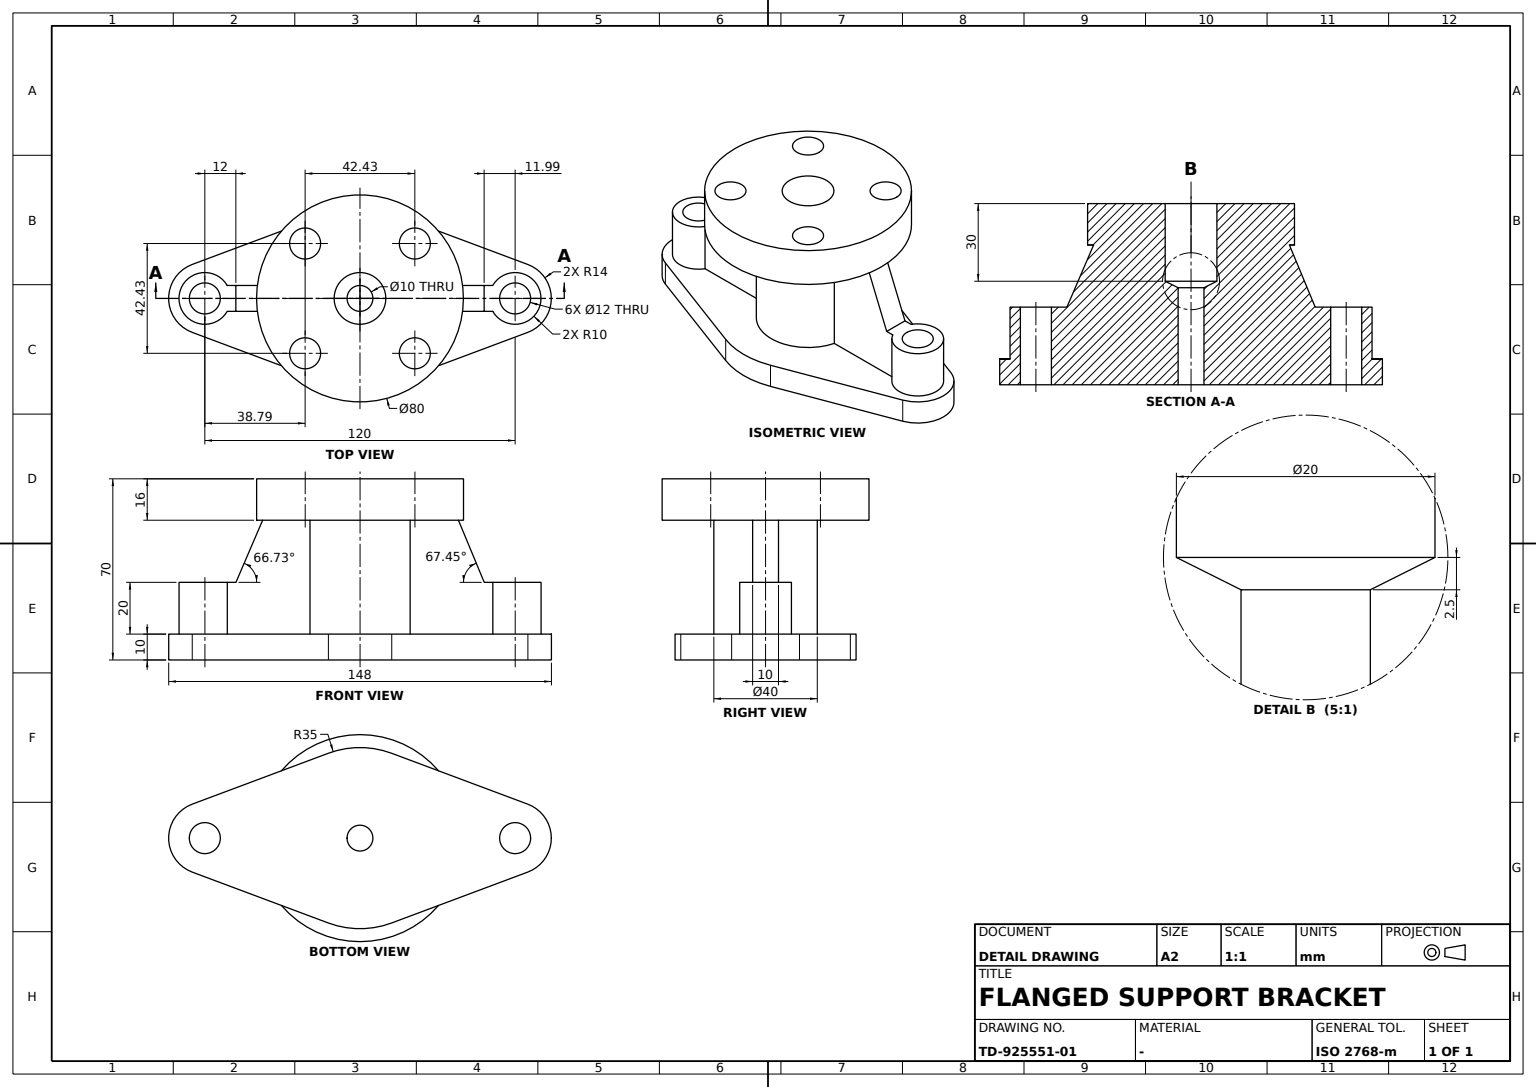
ISO-10303-21;
HEADER;
FILE_DESCRIPTION((''),'2;1');
FILE_NAME('','',(''),(''),'','','');
FILE_SCHEMA(('AUTOMOTIVE_DESIGN'));
ENDSEC;
DATA;
#1=APPLICATION_CONTEXT('');
#2=PRODUCT_CONTEXT('',#1,'mechanical');
#3=PRODUCT('','','',(#2));
#4=PRODUCT_DEFINITION_FORMATION('','',#3);
#5=PRODUCT_DEFINITION_CONTEXT('',#1,'design');
#6=PRODUCT_DEFINITION('','',#4,#5);
#7=PRODUCT_DEFINITION_SHAPE('','',#6);
#8=(LENGTH_UNIT()NAMED_UNIT(*)SI_UNIT(.MILLI.,.METRE.));
#9=(NAMED_UNIT(*)PLANE_ANGLE_UNIT()SI_UNIT($,.RADIAN.));
#10=(NAMED_UNIT(*)SI_UNIT($,.STERADIAN.)SOLID_ANGLE_UNIT());
#11=UNCERTAINTY_MEASURE_WITH_UNIT(LENGTH_MEASURE(1.E-05),#8,'distance_accuracy_value','');
#12=(GEOMETRIC_REPRESENTATION_CONTEXT(3)GLOBAL_UNCERTAINTY_ASSIGNED_CONTEXT((#11))GLOBAL_UNIT_ASSIGNED_CONTEXT((#8,#9,#10))REPRESENTATION_CONTEXT('',''));
#13=CARTESIAN_POINT('',(12.25,32.786239,10.));
#14=VERTEX_POINT('',#13);
#15=CARTESIAN_POINT('',(-12.25,32.786239,10.));
#16=VERTEX_POINT('',#15);
#17=CARTESIAN_POINT('',(0.,0.,10.));
#18=DIRECTION('',(0.,0.,1.));
#19=DIRECTION('',(1.,0.,0.));
#20=AXIS2_PLACEMENT_3D('',#17,#18,#19);
#21=CIRCLE('',#20,35.);
#22=EDGE_CURVE('',#14,#16,#21,.T.);
#23=ORIENTED_EDGE('',*,*,#22,.F.);
#24=CARTESIAN_POINT('',(12.25,32.786239,0.));
#25=VERTEX_POINT('',#24);
#26=CARTESIAN_POINT('',(12.25,32.786239,5.));
#27=VECTOR('',#18,1000.);
#28=LINE('',#26,#27);
#29=EDGE_CURVE('',#25,#14,#28,.T.);
#30=ORIENTED_EDGE('',*,*,#29,.F.);
#31=CARTESIAN_POINT('',(-12.25,32.786239,0.));
#32=VERTEX_POINT('',#31);
#33=CARTESIAN_POINT('',(0.,0.,0.));
#34=AXIS2_PLACEMENT_3D('',#33,#18,#19);
#35=CIRCLE('',#34,35.);
#36=EDGE_CURVE('',#25,#32,#35,.T.);
#37=ORIENTED_EDGE('',*,*,#36,.T.);
#38=CARTESIAN_POINT('',(-12.25,32.786239,5.));
#39=LINE('',#38,#27);
#40=EDGE_CURVE('',#32,#16,#39,.T.);
#41=ORIENTED_EDGE('',*,*,#40,.T.);
#42=EDGE_LOOP('',(#23,#30,#37,#41));
#43=FACE_OUTER_BOUND('',#42,.T.);
#44=CARTESIAN_POINT('',(0.,0.,5.));
#45=DIRECTION('',(0.,0.,-1.));
#46=AXIS2_PLACEMENT_3D('',#44,#45,#19);
#47=CYLINDRICAL_SURFACE('',#46,35.);
#48=ADVANCED_FACE('',(#43),#47,.T.);
#49=CARTESIAN_POINT('',(-37.677164,5.,54.));
#50=VERTEX_POINT('',#49);
#51=CARTESIAN_POINT('',(-19.364917,5.,54.));
#52=VERTEX_POINT('',#51);
#53=CARTESIAN_POINT('',(-28.52104,5.,54.));
#54=VECTOR('',#19,1000.);
#55=LINE('',#53,#54);
#56=EDGE_CURVE('',#50,#52,#55,.T.);
#57=ORIENTED_EDGE('',*,*,#56,.F.);
#58=CARTESIAN_POINT('',(-37.677164,-5.,54.));
#59=VERTEX_POINT('',#58);
#60=CARTESIAN_POINT('',(-37.677164,0.,54.));
#61=DIRECTION('',(0.,-1.,0.));
#62=VECTOR('',#61,1000.);
#63=LINE('',#60,#62);
#64=EDGE_CURVE('',#50,#59,#63,.T.);
#65=ORIENTED_EDGE('',*,*,#64,.T.);
#66=CARTESIAN_POINT('',(-19.364917,-5.,54.));
#67=VERTEX_POINT('',#66);
#68=CARTESIAN_POINT('',(-28.52104,-5.,54.));
#69=LINE('',#68,#54);
#70=EDGE_CURVE('',#59,#67,#69,.T.);
#71=ORIENTED_EDGE('',*,*,#70,.T.);
#72=CARTESIAN_POINT('',(19.364917,-5.,54.));
#73=VERTEX_POINT('',#72);
#74=CARTESIAN_POINT('',(0.,0.,54.));
#75=AXIS2_PLACEMENT_3D('',#74,#18,#19);
#76=CIRCLE('',#75,20.);
#77=EDGE_CURVE('',#67,#73,#76,.T.);
#78=ORIENTED_EDGE('',*,*,#77,.T.);
#79=CARTESIAN_POINT('',(38.044305,-5.,54.));
#80=VERTEX_POINT('',#79);
#81=CARTESIAN_POINT('',(28.704611,-5.,54.));
#82=LINE('',#81,#54);
#83=EDGE_CURVE('',#73,#80,#82,.T.);
#84=ORIENTED_EDGE('',*,*,#83,.T.);
#85=CARTESIAN_POINT('',(38.044305,5.,54.));
#86=VERTEX_POINT('',#85);
#87=CARTESIAN_POINT('',(38.044305,0.,54.));
#88=LINE('',#87,#62);
#89=EDGE_CURVE('',#86,#80,#88,.T.);
#90=ORIENTED_EDGE('',*,*,#89,.F.);
#91=CARTESIAN_POINT('',(19.364917,5.,54.));
#92=VERTEX_POINT('',#91);
#93=CARTESIAN_POINT('',(28.704611,5.,54.));
#94=LINE('',#93,#54);
#95=EDGE_CURVE('',#92,#86,#94,.T.);
#96=ORIENTED_EDGE('',*,*,#95,.F.);
#97=EDGE_CURVE('',#92,#52,#76,.T.);
#98=ORIENTED_EDGE('',*,*,#97,.T.);
#99=EDGE_LOOP('',(#57,#65,#71,#78,#84,#90,#96,#98));
#100=FACE_BOUND('',#99,.T.);
#101=CARTESIAN_POINT('',(-15.213203,-21.213203,54.));
#102=VERTEX_POINT('',#101);
#103=CARTESIAN_POINT('',(-27.213203,-21.213203,54.));
#104=VERTEX_POINT('',#103);
#105=CARTESIAN_POINT('',(-21.213203,-21.213203,54.));
#106=AXIS2_PLACEMENT_3D('',#105,#18,#19);
#107=CIRCLE('',#106,6.);
#108=EDGE_CURVE('',#102,#104,#107,.T.);
#109=ORIENTED_EDGE('',*,*,#108,.T.);
#110=EDGE_CURVE('',#104,#102,#107,.T.);
#111=ORIENTED_EDGE('',*,*,#110,.T.);
#112=EDGE_LOOP('',(#109,#111));
#113=FACE_BOUND('',#112,.T.);
#114=CARTESIAN_POINT('',(40.,0.,54.));
#115=VERTEX_POINT('',#114);
#116=CARTESIAN_POINT('',(-40.,0.,54.));
#117=VERTEX_POINT('',#116);
#118=CIRCLE('',#75,40.);
#119=EDGE_CURVE('',#115,#117,#118,.T.);
#120=ORIENTED_EDGE('',*,*,#119,.F.);
#121=EDGE_CURVE('',#117,#115,#118,.T.);
#122=ORIENTED_EDGE('',*,*,#121,.F.);
#123=EDGE_LOOP('',(#120,#122));
#124=FACE_OUTER_BOUND('',#123,.T.);
#125=CARTESIAN_POINT('',(15.213203,21.213203,54.));
#126=VERTEX_POINT('',#125);
#127=CARTESIAN_POINT('',(27.213203,21.213203,54.));
#128=VERTEX_POINT('',#127);
#129=CARTESIAN_POINT('',(21.213203,21.213203,54.));
#130=AXIS2_PLACEMENT_3D('',#129,#18,#19);
#131=CIRCLE('',#130,6.);
#132=EDGE_CURVE('',#126,#128,#131,.T.);
#133=ORIENTED_EDGE('',*,*,#132,.T.);
#134=EDGE_CURVE('',#128,#126,#131,.T.);
#135=ORIENTED_EDGE('',*,*,#134,.T.);
#136=EDGE_LOOP('',(#133,#135));
#137=FACE_BOUND('',#136,.T.);
#138=CARTESIAN_POINT('',(-27.213203,21.213203,54.));
#139=VERTEX_POINT('',#138);
#140=CARTESIAN_POINT('',(-15.213203,21.213203,54.));
#141=VERTEX_POINT('',#140);
#142=CARTESIAN_POINT('',(-21.213203,21.213203,54.));
#143=AXIS2_PLACEMENT_3D('',#142,#18,#19);
#144=CIRCLE('',#143,6.);
#145=EDGE_CURVE('',#139,#141,#144,.T.);
#146=ORIENTED_EDGE('',*,*,#145,.T.);
#147=EDGE_CURVE('',#141,#139,#144,.T.);
#148=ORIENTED_EDGE('',*,*,#147,.T.);
#149=EDGE_LOOP('',(#146,#148));
#150=FACE_BOUND('',#149,.T.);
#151=CARTESIAN_POINT('',(27.213203,-21.213203,54.));
#152=VERTEX_POINT('',#151);
#153=CARTESIAN_POINT('',(15.213203,-21.213203,54.));
#154=VERTEX_POINT('',#153);
#155=CARTESIAN_POINT('',(21.213203,-21.213203,54.));
#156=AXIS2_PLACEMENT_3D('',#155,#18,#19);
#157=CIRCLE('',#156,6.);
#158=EDGE_CURVE('',#152,#154,#157,.T.);
#159=ORIENTED_EDGE('',*,*,#158,.T.);
#160=EDGE_CURVE('',#154,#152,#157,.T.);
#161=ORIENTED_EDGE('',*,*,#160,.T.);
#162=EDGE_LOOP('',(#159,#161));
#163=FACE_BOUND('',#162,.T.);
#164=PLANE('',#75);
#165=ADVANCED_FACE('',(#100,#113,#124,#137,#150,#163),#164,.F.);
#166=CARTESIAN_POINT('',(64.9,13.114496,0.));
#167=VERTEX_POINT('',#166);
#168=CARTESIAN_POINT('',(64.9,13.114496,10.));
#169=VERTEX_POINT('',#168);
#170=CARTESIAN_POINT('',(64.9,13.114496,5.));
#171=LINE('',#170,#27);
#172=EDGE_CURVE('',#167,#169,#171,.T.);
#173=ORIENTED_EDGE('',*,*,#172,.T.);
#174=CARTESIAN_POINT('',(74.,0.,10.));
#175=VERTEX_POINT('',#174);
#176=CARTESIAN_POINT('',(60.,0.,10.));
#177=AXIS2_PLACEMENT_3D('',#176,#18,#19);
#178=CIRCLE('',#177,14.);
#179=EDGE_CURVE('',#175,#169,#178,.T.);
#180=ORIENTED_EDGE('',*,*,#179,.F.);
#181=CARTESIAN_POINT('',(74.,0.,0.));
#182=VERTEX_POINT('',#181);
#183=CARTESIAN_POINT('',(74.,0.,5.));
#184=VECTOR('',#45,1000.);
#185=LINE('',#183,#184);
#186=EDGE_CURVE('',#175,#182,#185,.T.);
#187=ORIENTED_EDGE('',*,*,#186,.T.);
#188=CARTESIAN_POINT('',(60.,0.,0.));
#189=AXIS2_PLACEMENT_3D('',#188,#18,#19);
#190=CIRCLE('',#189,14.);
#191=EDGE_CURVE('',#182,#167,#190,.T.);
#192=ORIENTED_EDGE('',*,*,#191,.T.);
#193=EDGE_LOOP('',(#173,#180,#187,#192));
#194=FACE_OUTER_BOUND('',#193,.T.);
#195=CARTESIAN_POINT('',(60.,0.,5.));
#196=AXIS2_PLACEMENT_3D('',#195,#45,#19);
#197=CYLINDRICAL_SURFACE('',#196,14.);
#198=ADVANCED_FACE('',(#194),#197,.T.);
#199=ORIENTED_EDGE('',*,*,#29,.T.);
#200=CARTESIAN_POINT('',(38.575,22.950368,10.));
#201=DIRECTION('',(-0.9367497,0.35,0.));
#202=VECTOR('',#201,1000.);
#203=LINE('',#200,#202);
#204=EDGE_CURVE('',#169,#14,#203,.T.);
#205=ORIENTED_EDGE('',*,*,#204,.F.);
#206=ORIENTED_EDGE('',*,*,#172,.F.);
#207=CARTESIAN_POINT('',(38.575,22.950368,0.));
#208=LINE('',#207,#202);
#209=EDGE_CURVE('',#167,#25,#208,.T.);
#210=ORIENTED_EDGE('',*,*,#209,.T.);
#211=EDGE_LOOP('',(#199,#205,#206,#210));
#212=FACE_OUTER_BOUND('',#211,.T.);
#213=DIRECTION('',(-0.35,-0.9367497,0.));
#214=DIRECTION('',(0.9367497,-0.35,0.));
#215=AXIS2_PLACEMENT_3D('',#24,#213,#214);
#216=PLANE('',#215);
#217=ADVANCED_FACE('',(#212),#216,.F.);
#218=CARTESIAN_POINT('',(-12.25,-32.786239,0.));
#219=VERTEX_POINT('',#218);
#220=CARTESIAN_POINT('',(-12.25,-32.786239,10.));
#221=VERTEX_POINT('',#220);
#222=CARTESIAN_POINT('',(-12.25,-32.786239,5.));
#223=LINE('',#222,#27);
#224=EDGE_CURVE('',#219,#221,#223,.T.);
#225=ORIENTED_EDGE('',*,*,#224,.F.);
#226=CARTESIAN_POINT('',(12.25,-32.786239,0.));
#227=VERTEX_POINT('',#226);
#228=EDGE_CURVE('',#219,#227,#35,.T.);
#229=ORIENTED_EDGE('',*,*,#228,.T.);
#230=CARTESIAN_POINT('',(12.25,-32.786239,10.));
#231=VERTEX_POINT('',#230);
#232=CARTESIAN_POINT('',(12.25,-32.786239,5.));
#233=LINE('',#232,#27);
#234=EDGE_CURVE('',#227,#231,#233,.T.);
#235=ORIENTED_EDGE('',*,*,#234,.T.);
#236=EDGE_CURVE('',#221,#231,#21,.T.);
#237=ORIENTED_EDGE('',*,*,#236,.F.);
#238=EDGE_LOOP('',(#225,#229,#235,#237));
#239=FACE_OUTER_BOUND('',#238,.T.);
#240=ADVANCED_FACE('',(#239),#47,.T.);
#241=CARTESIAN_POINT('',(-64.9,-13.114496,10.));
#242=VERTEX_POINT('',#241);
#243=CARTESIAN_POINT('',(-38.575,-22.950368,10.));
#244=VECTOR('',#214,1000.);
#245=LINE('',#243,#244);
#246=EDGE_CURVE('',#242,#221,#245,.T.);
#247=ORIENTED_EDGE('',*,*,#246,.F.);
#248=CARTESIAN_POINT('',(-64.9,-13.114496,0.));
#249=VERTEX_POINT('',#248);
#250=CARTESIAN_POINT('',(-64.9,-13.114496,5.));
#251=LINE('',#250,#27);
#252=EDGE_CURVE('',#249,#242,#251,.T.);
#253=ORIENTED_EDGE('',*,*,#252,.F.);
#254=CARTESIAN_POINT('',(-38.575,-22.950368,0.));
#255=LINE('',#254,#244);
#256=EDGE_CURVE('',#249,#219,#255,.T.);
#257=ORIENTED_EDGE('',*,*,#256,.T.);
#258=ORIENTED_EDGE('',*,*,#224,.T.);
#259=EDGE_LOOP('',(#247,#253,#257,#258));
#260=FACE_OUTER_BOUND('',#259,.T.);
#261=AXIS2_PLACEMENT_3D('',#248,#213,#214);
#262=PLANE('',#261);
#263=ADVANCED_FACE('',(#260),#262,.T.);
#264=CARTESIAN_POINT('',(51.339746,5.,10.));
#265=VERTEX_POINT('',#264);
#266=CARTESIAN_POINT('',(51.339746,5.,30.));
#267=VERTEX_POINT('',#266);
#268=CARTESIAN_POINT('',(51.339746,5.,20.));
#269=LINE('',#268,#27);
#270=EDGE_CURVE('',#265,#267,#269,.T.);
#271=ORIENTED_EDGE('',*,*,#270,.T.);
#272=CARTESIAN_POINT('',(70.,0.,30.));
#273=VERTEX_POINT('',#272);
#274=CARTESIAN_POINT('',(60.,0.,30.));
#275=AXIS2_PLACEMENT_3D('',#274,#18,#19);
#276=CIRCLE('',#275,10.);
#277=EDGE_CURVE('',#273,#267,#276,.T.);
#278=ORIENTED_EDGE('',*,*,#277,.F.);
#279=CARTESIAN_POINT('',(70.,0.,10.));
#280=VERTEX_POINT('',#279);
#281=CARTESIAN_POINT('',(70.,0.,20.));
#282=LINE('',#281,#27);
#283=EDGE_CURVE('',#280,#273,#282,.T.);
#284=ORIENTED_EDGE('',*,*,#283,.F.);
#285=CIRCLE('',#177,10.);
#286=EDGE_CURVE('',#280,#265,#285,.T.);
#287=ORIENTED_EDGE('',*,*,#286,.T.);
#288=EDGE_LOOP('',(#271,#278,#284,#287));
#289=FACE_OUTER_BOUND('',#288,.T.);
#290=CARTESIAN_POINT('',(60.,0.,20.));
#291=AXIS2_PLACEMENT_3D('',#290,#45,#19);
#292=CYLINDRICAL_SURFACE('',#291,10.);
#293=ADVANCED_FACE('',(#289),#292,.T.);
#294=CARTESIAN_POINT('',(-64.9,13.114496,0.));
#295=VERTEX_POINT('',#294);
#296=CARTESIAN_POINT('',(-64.9,13.114496,10.));
#297=VERTEX_POINT('',#296);
#298=CARTESIAN_POINT('',(-64.9,13.114496,5.));
#299=LINE('',#298,#27);
#300=EDGE_CURVE('',#295,#297,#299,.T.);
#301=ORIENTED_EDGE('',*,*,#300,.F.);
#302=CARTESIAN_POINT('',(-60.,0.,0.));
#303=AXIS2_PLACEMENT_3D('',#302,#18,#19);
#304=CIRCLE('',#303,14.);
#305=EDGE_CURVE('',#295,#249,#304,.T.);
#306=ORIENTED_EDGE('',*,*,#305,.T.);
#307=ORIENTED_EDGE('',*,*,#252,.T.);
#308=CARTESIAN_POINT('',(-60.,0.,10.));
#309=AXIS2_PLACEMENT_3D('',#308,#18,#19);
#310=CIRCLE('',#309,14.);
#311=EDGE_CURVE('',#297,#242,#310,.T.);
#312=ORIENTED_EDGE('',*,*,#311,.F.);
#313=EDGE_LOOP('',(#301,#306,#307,#312));
#314=FACE_OUTER_BOUND('',#313,.T.);
#315=CARTESIAN_POINT('',(-60.,0.,5.));
#316=AXIS2_PLACEMENT_3D('',#315,#45,#19);
#317=CYLINDRICAL_SURFACE('',#316,14.);
#318=ADVANCED_FACE('',(#314),#317,.T.);
#319=CARTESIAN_POINT('',(50.277016,-5.,30.));
#320=VERTEX_POINT('',#319);
#321=CARTESIAN_POINT('',(50.277016,5.,30.));
#322=VERTEX_POINT('',#321);
#323=CARTESIAN_POINT('',(50.277016,0.,30.));
#324=DIRECTION('',(0.,1.,0.));
#325=VECTOR('',#324,1000.);
#326=LINE('',#323,#325);
#327=EDGE_CURVE('',#320,#322,#326,.T.);
#328=ORIENTED_EDGE('',*,*,#327,.T.);
#329=CARTESIAN_POINT('',(48.011559,5.,30.));
#330=VERTEX_POINT('',#329);
#331=CARTESIAN_POINT('',(49.144287,5.,30.));
#332=DIRECTION('',(-1.,0.,0.));
#333=VECTOR('',#332,1000.);
#334=LINE('',#331,#333);
#335=EDGE_CURVE('',#322,#330,#334,.T.);
#336=ORIENTED_EDGE('',*,*,#335,.T.);
#337=CARTESIAN_POINT('',(48.011559,-5.,30.));
#338=VERTEX_POINT('',#337);
#339=CARTESIAN_POINT('',(48.011559,0.,30.));
#340=LINE('',#339,#325);
#341=EDGE_CURVE('',#338,#330,#340,.T.);
#342=ORIENTED_EDGE('',*,*,#341,.F.);
#343=CARTESIAN_POINT('',(49.144287,-5.,30.));
#344=LINE('',#343,#333);
#345=EDGE_CURVE('',#320,#338,#344,.T.);
#346=ORIENTED_EDGE('',*,*,#345,.F.);
#347=EDGE_LOOP('',(#328,#336,#342,#346));
#348=FACE_OUTER_BOUND('',#347,.T.);
#349=CARTESIAN_POINT('',(0.,0.,30.));
#350=AXIS2_PLACEMENT_3D('',#349,#18,#19);
#351=PLANE('',#350);
#352=ADVANCED_FACE('',(#348),#351,.T.);
#353=ORIENTED_EDGE('',*,*,#121,.T.);
#354=CARTESIAN_POINT('',(40.,0.,70.));
#355=VERTEX_POINT('',#354);
#356=CARTESIAN_POINT('',(40.,0.,62.));
#357=LINE('',#356,#27);
#358=EDGE_CURVE('',#115,#355,#357,.T.);
#359=ORIENTED_EDGE('',*,*,#358,.T.);
#360=CARTESIAN_POINT('',(-40.,0.,70.));
#361=VERTEX_POINT('',#360);
#362=CARTESIAN_POINT('',(0.,0.,70.));
#363=AXIS2_PLACEMENT_3D('',#362,#18,#19);
#364=CIRCLE('',#363,40.);
#365=EDGE_CURVE('',#361,#355,#364,.T.);
#366=ORIENTED_EDGE('',*,*,#365,.F.);
#367=CARTESIAN_POINT('',(-40.,0.,62.));
#368=LINE('',#367,#27);
#369=EDGE_CURVE('',#117,#361,#368,.T.);
#370=ORIENTED_EDGE('',*,*,#369,.F.);
#371=EDGE_LOOP('',(#353,#359,#366,#370));
#372=FACE_OUTER_BOUND('',#371,.T.);
#373=CARTESIAN_POINT('',(0.,0.,62.));
#374=AXIS2_PLACEMENT_3D('',#373,#45,#19);
#375=CYLINDRICAL_SURFACE('',#374,40.);
#376=ADVANCED_FACE('',(#372),#375,.T.);
#377=CARTESIAN_POINT('',(-15.213203,-21.213203,70.));
#378=VERTEX_POINT('',#377);
#379=CARTESIAN_POINT('',(-15.213203,-21.213203,62.));
#380=LINE('',#379,#184);
#381=EDGE_CURVE('',#378,#102,#380,.T.);
#382=ORIENTED_EDGE('',*,*,#381,.T.);
#383=ORIENTED_EDGE('',*,*,#110,.F.);
#384=CARTESIAN_POINT('',(-27.213203,-21.213203,70.));
#385=VERTEX_POINT('',#384);
#386=CARTESIAN_POINT('',(-27.213203,-21.213203,62.));
#387=LINE('',#386,#184);
#388=EDGE_CURVE('',#385,#104,#387,.T.);
#389=ORIENTED_EDGE('',*,*,#388,.F.);
#390=CARTESIAN_POINT('',(-21.213203,-21.213203,70.));
#391=AXIS2_PLACEMENT_3D('',#390,#18,#19);
#392=CIRCLE('',#391,6.);
#393=EDGE_CURVE('',#385,#378,#392,.T.);
#394=ORIENTED_EDGE('',*,*,#393,.T.);
#395=EDGE_LOOP('',(#382,#383,#389,#394));
#396=FACE_OUTER_BOUND('',#395,.T.);
#397=CARTESIAN_POINT('',(-21.213203,-21.213203,62.));
#398=AXIS2_PLACEMENT_3D('',#397,#45,#19);
#399=CYLINDRICAL_SURFACE('',#398,6.);
#400=ADVANCED_FACE('',(#396),#399,.F.);
#401=CARTESIAN_POINT('',(5.,0.,37.5));
#402=VERTEX_POINT('',#401);
#403=CARTESIAN_POINT('',(10.,0.,40.));
#404=VERTEX_POINT('',#403);
#405=CARTESIAN_POINT('',(7.5,0.,38.75));
#406=DIRECTION('',(0.894427191,0.,0.447213595));
#407=VECTOR('',#406,1000.);
#408=LINE('',#405,#407);
#409=EDGE_CURVE('',#402,#404,#408,.T.);
#410=ORIENTED_EDGE('',*,*,#409,.F.);
#411=CARTESIAN_POINT('',(-5.,0.,37.5));
#412=VERTEX_POINT('',#411);
#413=CARTESIAN_POINT('',(0.,0.,37.5));
#414=AXIS2_PLACEMENT_3D('',#413,#18,#19);
#415=CIRCLE('',#414,5.);
#416=EDGE_CURVE('',#412,#402,#415,.T.);
#417=ORIENTED_EDGE('',*,*,#416,.F.);
#418=CARTESIAN_POINT('',(-10.,0.,40.));
#419=VERTEX_POINT('',#418);
#420=CARTESIAN_POINT('',(-7.5,0.,38.75));
#421=DIRECTION('',(-0.894427191,0.,0.447213595));
#422=VECTOR('',#421,1000.);
#423=LINE('',#420,#422);
#424=EDGE_CURVE('',#412,#419,#423,.T.);
#425=ORIENTED_EDGE('',*,*,#424,.T.);
#426=CARTESIAN_POINT('',(0.,0.,40.));
#427=AXIS2_PLACEMENT_3D('',#426,#45,#19);
#428=CIRCLE('',#427,10.);
#429=EDGE_CURVE('',#404,#419,#428,.T.);
#430=ORIENTED_EDGE('',*,*,#429,.F.);
#431=EDGE_LOOP('',(#410,#417,#425,#430));
#432=FACE_OUTER_BOUND('',#431,.T.);
#433=CONICAL_SURFACE('',#414,5.,1.107148718);
#434=ADVANCED_FACE('',(#432),#433,.F.);
#435=CARTESIAN_POINT('',(64.9,-13.114496,0.));
#436=VERTEX_POINT('',#435);
#437=CARTESIAN_POINT('',(38.575,-22.950368,0.));
#438=DIRECTION('',(0.9367497,0.35,0.));
#439=VECTOR('',#438,1000.);
#440=LINE('',#437,#439);
#441=EDGE_CURVE('',#227,#436,#440,.T.);
#442=ORIENTED_EDGE('',*,*,#441,.T.);
#443=CARTESIAN_POINT('',(64.9,-13.114496,10.));
#444=VERTEX_POINT('',#443);
#445=CARTESIAN_POINT('',(64.9,-13.114496,5.));
#446=LINE('',#445,#27);
#447=EDGE_CURVE('',#436,#444,#446,.T.);
#448=ORIENTED_EDGE('',*,*,#447,.T.);
#449=CARTESIAN_POINT('',(38.575,-22.950368,10.));
#450=LINE('',#449,#439);
#451=EDGE_CURVE('',#231,#444,#450,.T.);
#452=ORIENTED_EDGE('',*,*,#451,.F.);
#453=ORIENTED_EDGE('',*,*,#234,.F.);
#454=EDGE_LOOP('',(#442,#448,#452,#453));
#455=FACE_OUTER_BOUND('',#454,.T.);
#456=DIRECTION('',(0.35,-0.9367497,0.));
#457=AXIS2_PLACEMENT_3D('',#226,#456,#438);
#458=PLANE('',#457);
#459=ADVANCED_FACE('',(#455),#458,.T.);
#460=CARTESIAN_POINT('',(-70.,0.,10.));
#461=VERTEX_POINT('',#460);
#462=CARTESIAN_POINT('',(-51.339746,-5.,10.));
#463=VERTEX_POINT('',#462);
#464=CIRCLE('',#309,10.);
#465=EDGE_CURVE('',#461,#463,#464,.T.);
#466=ORIENTED_EDGE('',*,*,#465,.T.);
#467=CARTESIAN_POINT('',(-51.339746,-5.,30.));
#468=VERTEX_POINT('',#467);
#469=CARTESIAN_POINT('',(-51.339746,-5.,20.));
#470=LINE('',#469,#27);
#471=EDGE_CURVE('',#463,#468,#470,.T.);
#472=ORIENTED_EDGE('',*,*,#471,.T.);
#473=CARTESIAN_POINT('',(-70.,0.,30.));
#474=VERTEX_POINT('',#473);
#475=CARTESIAN_POINT('',(-60.,0.,30.));
#476=AXIS2_PLACEMENT_3D('',#475,#18,#19);
#477=CIRCLE('',#476,10.);
#478=EDGE_CURVE('',#474,#468,#477,.T.);
#479=ORIENTED_EDGE('',*,*,#478,.F.);
#480=CARTESIAN_POINT('',(-70.,0.,20.));
#481=LINE('',#480,#27);
#482=EDGE_CURVE('',#461,#474,#481,.T.);
#483=ORIENTED_EDGE('',*,*,#482,.F.);
#484=EDGE_LOOP('',(#466,#472,#479,#483));
#485=FACE_OUTER_BOUND('',#484,.T.);
#486=CARTESIAN_POINT('',(-60.,0.,20.));
#487=AXIS2_PLACEMENT_3D('',#486,#45,#19);
#488=CYLINDRICAL_SURFACE('',#487,10.);
#489=ADVANCED_FACE('',(#485),#488,.T.);
#490=CARTESIAN_POINT('',(54.,0.,0.));
#491=VERTEX_POINT('',#490);
#492=CARTESIAN_POINT('',(66.,0.,0.));
#493=VERTEX_POINT('',#492);
#494=CIRCLE('',#189,6.);
#495=EDGE_CURVE('',#491,#493,#494,.T.);
#496=ORIENTED_EDGE('',*,*,#495,.T.);
#497=EDGE_CURVE('',#493,#491,#494,.T.);
#498=ORIENTED_EDGE('',*,*,#497,.T.);
#499=EDGE_LOOP('',(#496,#498));
#500=FACE_BOUND('',#499,.T.);
#501=CARTESIAN_POINT('',(-5.,0.,0.));
#502=VERTEX_POINT('',#501);
#503=CARTESIAN_POINT('',(5.,0.,0.));
#504=VERTEX_POINT('',#503);
#505=AXIS2_PLACEMENT_3D('',#33,#45,#19);
#506=CIRCLE('',#505,5.);
#507=EDGE_CURVE('',#502,#504,#506,.T.);
#508=ORIENTED_EDGE('',*,*,#507,.F.);
#509=EDGE_CURVE('',#504,#502,#506,.T.);
#510=ORIENTED_EDGE('',*,*,#509,.F.);
#511=EDGE_LOOP('',(#508,#510));
#512=FACE_BOUND('',#511,.T.);
#513=CARTESIAN_POINT('',(-66.,0.,0.));
#514=VERTEX_POINT('',#513);
#515=CARTESIAN_POINT('',(-54.,0.,0.));
#516=VERTEX_POINT('',#515);
#517=CIRCLE('',#303,6.);
#518=EDGE_CURVE('',#514,#516,#517,.T.);
#519=ORIENTED_EDGE('',*,*,#518,.T.);
#520=EDGE_CURVE('',#516,#514,#517,.T.);
#521=ORIENTED_EDGE('',*,*,#520,.T.);
#522=EDGE_LOOP('',(#519,#521));
#523=FACE_BOUND('',#522,.T.);
#524=EDGE_CURVE('',#436,#182,#190,.T.);
#525=ORIENTED_EDGE('',*,*,#524,.F.);
#526=ORIENTED_EDGE('',*,*,#441,.F.);
#527=ORIENTED_EDGE('',*,*,#228,.F.);
#528=ORIENTED_EDGE('',*,*,#256,.F.);
#529=ORIENTED_EDGE('',*,*,#305,.F.);
#530=CARTESIAN_POINT('',(-38.575,22.950368,0.));
#531=DIRECTION('',(-0.9367497,-0.35,0.));
#532=VECTOR('',#531,1000.);
#533=LINE('',#530,#532);
#534=EDGE_CURVE('',#32,#295,#533,.T.);
#535=ORIENTED_EDGE('',*,*,#534,.F.);
#536=ORIENTED_EDGE('',*,*,#36,.F.);
#537=ORIENTED_EDGE('',*,*,#209,.F.);
#538=ORIENTED_EDGE('',*,*,#191,.F.);
#539=EDGE_LOOP('',(#525,#526,#527,#528,#529,#535,#536,#537,#538));
#540=FACE_OUTER_BOUND('',#539,.T.);
#541=PLANE('',#34);
#542=ADVANCED_FACE('',(#500,#512,#523,#540),#541,.F.);
#543=ORIENTED_EDGE('',*,*,#369,.T.);
#544=EDGE_CURVE('',#355,#361,#364,.T.);
#545=ORIENTED_EDGE('',*,*,#544,.F.);
#546=ORIENTED_EDGE('',*,*,#358,.F.);
#547=ORIENTED_EDGE('',*,*,#119,.T.);
#548=EDGE_LOOP('',(#543,#545,#546,#547));
#549=FACE_OUTER_BOUND('',#548,.T.);
#550=ADVANCED_FACE('',(#549),#375,.T.);
#551=CARTESIAN_POINT('',(54.,0.,30.));
#552=VERTEX_POINT('',#551);
#553=CARTESIAN_POINT('',(66.,0.,30.));
#554=VERTEX_POINT('',#553);
#555=CIRCLE('',#275,6.);
#556=EDGE_CURVE('',#552,#554,#555,.T.);
#557=ORIENTED_EDGE('',*,*,#556,.T.);
#558=CARTESIAN_POINT('',(66.,0.,14.34));
#559=LINE('',#558,#184);
#560=EDGE_CURVE('',#554,#493,#559,.T.);
#561=ORIENTED_EDGE('',*,*,#560,.T.);
#562=ORIENTED_EDGE('',*,*,#495,.F.);
#563=CARTESIAN_POINT('',(54.,0.,14.34));
#564=LINE('',#563,#184);
#565=EDGE_CURVE('',#552,#491,#564,.T.);
#566=ORIENTED_EDGE('',*,*,#565,.F.);
#567=EDGE_LOOP('',(#557,#561,#562,#566));
#568=FACE_OUTER_BOUND('',#567,.T.);
#569=CARTESIAN_POINT('',(60.,0.,14.34));
#570=AXIS2_PLACEMENT_3D('',#569,#45,#19);
#571=CYLINDRICAL_SURFACE('',#570,6.);
#572=ADVANCED_FACE('',(#568),#571,.F.);
#573=ORIENTED_EDGE('',*,*,#97,.F.);
#574=CARTESIAN_POINT('',(19.364917,5.,10.));
#575=VERTEX_POINT('',#574);
#576=CARTESIAN_POINT('',(19.364917,5.,32.));
#577=LINE('',#576,#27);
#578=EDGE_CURVE('',#575,#92,#577,.T.);
#579=ORIENTED_EDGE('',*,*,#578,.F.);
#580=CARTESIAN_POINT('',(-19.364917,5.,10.));
#581=VERTEX_POINT('',#580);
#582=CIRCLE('',#20,20.);
#583=EDGE_CURVE('',#575,#581,#582,.T.);
#584=ORIENTED_EDGE('',*,*,#583,.T.);
#585=CARTESIAN_POINT('',(-19.364917,5.,32.));
#586=LINE('',#585,#27);
#587=EDGE_CURVE('',#581,#52,#586,.T.);
#588=ORIENTED_EDGE('',*,*,#587,.T.);
#589=EDGE_LOOP('',(#573,#579,#584,#588));
#590=FACE_OUTER_BOUND('',#589,.T.);
#591=CARTESIAN_POINT('',(0.,0.,32.));
#592=AXIS2_PLACEMENT_3D('',#591,#45,#19);
#593=CYLINDRICAL_SURFACE('',#592,20.);
#594=ADVANCED_FACE('',(#590),#593,.T.);
#595=CARTESIAN_POINT('',(19.364917,-5.,10.));
#596=VERTEX_POINT('',#595);
#597=CARTESIAN_POINT('',(19.364917,-5.,32.));
#598=LINE('',#597,#27);
#599=EDGE_CURVE('',#596,#73,#598,.T.);
#600=ORIENTED_EDGE('',*,*,#599,.F.);
#601=CARTESIAN_POINT('',(51.339746,-5.,10.));
#602=VERTEX_POINT('',#601);
#603=CARTESIAN_POINT('',(35.352331,-5.,10.));
#604=LINE('',#603,#54);
#605=EDGE_CURVE('',#596,#602,#604,.T.);
#606=ORIENTED_EDGE('',*,*,#605,.T.);
#607=CARTESIAN_POINT('',(51.339746,-5.,30.));
#608=VERTEX_POINT('',#607);
#609=CARTESIAN_POINT('',(51.339746,-5.,20.));
#610=LINE('',#609,#27);
#611=EDGE_CURVE('',#602,#608,#610,.T.);
#612=ORIENTED_EDGE('',*,*,#611,.T.);
#613=CARTESIAN_POINT('',(50.808381,-5.,30.));
#614=LINE('',#613,#333);
#615=EDGE_CURVE('',#608,#320,#614,.T.);
#616=ORIENTED_EDGE('',*,*,#615,.T.);
#617=ORIENTED_EDGE('',*,*,#345,.T.);
#618=CARTESIAN_POINT('',(43.027932,-5.,42.));
#619=DIRECTION('',(-0.383541444,0.,0.923523665));
#620=VECTOR('',#619,1000.);
#621=LINE('',#618,#620);
#622=EDGE_CURVE('',#338,#80,#621,.T.);
#623=ORIENTED_EDGE('',*,*,#622,.T.);
#624=ORIENTED_EDGE('',*,*,#83,.F.);
#625=EDGE_LOOP('',(#600,#606,#612,#616,#617,#623,#624));
#626=FACE_OUTER_BOUND('',#625,.T.);
#627=CARTESIAN_POINT('',(0.,-5.,0.));
#628=AXIS2_PLACEMENT_3D('',#627,#324,#332);
#629=PLANE('',#628);
#630=ADVANCED_FACE('',(#626),#629,.F.);
#631=CARTESIAN_POINT('',(-10.,0.,70.));
#632=VERTEX_POINT('',#631);
#633=CARTESIAN_POINT('',(-10.,0.,35.155));
#634=LINE('',#633,#27);
#635=EDGE_CURVE('',#419,#632,#634,.T.);
#636=ORIENTED_EDGE('',*,*,#635,.T.);
#637=CARTESIAN_POINT('',(10.,0.,70.));
#638=VERTEX_POINT('',#637);
#639=CIRCLE('',#363,10.);
#640=EDGE_CURVE('',#632,#638,#639,.T.);
#641=ORIENTED_EDGE('',*,*,#640,.T.);
#642=CARTESIAN_POINT('',(10.,0.,35.155));
#643=LINE('',#642,#27);
#644=EDGE_CURVE('',#404,#638,#643,.T.);
#645=ORIENTED_EDGE('',*,*,#644,.F.);
#646=ORIENTED_EDGE('',*,*,#429,.T.);
#647=EDGE_LOOP('',(#636,#641,#645,#646));
#648=FACE_OUTER_BOUND('',#647,.T.);
#649=CYLINDRICAL_SURFACE('',#363,10.);
#650=ADVANCED_FACE('',(#648),#649,.F.);
#651=CARTESIAN_POINT('',(-19.364917,-5.,10.));
#652=VERTEX_POINT('',#651);
#653=CARTESIAN_POINT('',(-19.364917,-5.,32.));
#654=LINE('',#653,#27);
#655=EDGE_CURVE('',#652,#67,#654,.T.);
#656=ORIENTED_EDGE('',*,*,#655,.F.);
#657=EDGE_CURVE('',#652,#596,#582,.T.);
#658=ORIENTED_EDGE('',*,*,#657,.T.);
#659=ORIENTED_EDGE('',*,*,#599,.T.);
#660=ORIENTED_EDGE('',*,*,#77,.F.);
#661=EDGE_LOOP('',(#656,#658,#659,#660));
#662=FACE_OUTER_BOUND('',#661,.T.);
#663=ADVANCED_FACE('',(#662),#593,.T.);
#664=ORIENTED_EDGE('',*,*,#108,.F.);
#665=ORIENTED_EDGE('',*,*,#381,.F.);
#666=EDGE_CURVE('',#378,#385,#392,.T.);
#667=ORIENTED_EDGE('',*,*,#666,.T.);
#668=ORIENTED_EDGE('',*,*,#388,.T.);
#669=EDGE_LOOP('',(#664,#665,#667,#668));
#670=FACE_OUTER_BOUND('',#669,.T.);
#671=ADVANCED_FACE('',(#670),#399,.F.);
#672=CARTESIAN_POINT('',(15.213203,21.213203,70.));
#673=VERTEX_POINT('',#672);
#674=CARTESIAN_POINT('',(27.213203,21.213203,70.));
#675=VERTEX_POINT('',#674);
#676=CARTESIAN_POINT('',(21.213203,21.213203,70.));
#677=AXIS2_PLACEMENT_3D('',#676,#18,#19);
#678=CIRCLE('',#677,6.);
#679=EDGE_CURVE('',#673,#675,#678,.T.);
#680=ORIENTED_EDGE('',*,*,#679,.T.);
#681=CARTESIAN_POINT('',(27.213203,21.213203,62.));
#682=LINE('',#681,#184);
#683=EDGE_CURVE('',#675,#128,#682,.T.);
#684=ORIENTED_EDGE('',*,*,#683,.T.);
#685=ORIENTED_EDGE('',*,*,#132,.F.);
#686=CARTESIAN_POINT('',(15.213203,21.213203,62.));
#687=LINE('',#686,#184);
#688=EDGE_CURVE('',#673,#126,#687,.T.);
#689=ORIENTED_EDGE('',*,*,#688,.F.);
#690=EDGE_LOOP('',(#680,#684,#685,#689));
#691=FACE_OUTER_BOUND('',#690,.T.);
#692=CARTESIAN_POINT('',(21.213203,21.213203,62.));
#693=AXIS2_PLACEMENT_3D('',#692,#45,#19);
#694=CYLINDRICAL_SURFACE('',#693,6.);
#695=ADVANCED_FACE('',(#691),#694,.F.);
#696=EDGE_CURVE('',#402,#412,#415,.T.);
#697=ORIENTED_EDGE('',*,*,#696,.F.);
#698=ORIENTED_EDGE('',*,*,#409,.T.);
#699=EDGE_CURVE('',#419,#404,#428,.T.);
#700=ORIENTED_EDGE('',*,*,#699,.F.);
#701=ORIENTED_EDGE('',*,*,#424,.F.);
#702=EDGE_LOOP('',(#697,#698,#700,#701));
#703=FACE_OUTER_BOUND('',#702,.T.);
#704=ADVANCED_FACE('',(#703),#433,.F.);
#705=ORIENTED_EDGE('',*,*,#236,.T.);
#706=ORIENTED_EDGE('',*,*,#451,.T.);
#707=EDGE_CURVE('',#444,#175,#178,.T.);
#708=ORIENTED_EDGE('',*,*,#707,.T.);
#709=ORIENTED_EDGE('',*,*,#179,.T.);
#710=ORIENTED_EDGE('',*,*,#204,.T.);
#711=ORIENTED_EDGE('',*,*,#22,.T.);
#712=CARTESIAN_POINT('',(-38.575,22.950368,10.));
#713=LINE('',#712,#532);
#714=EDGE_CURVE('',#16,#297,#713,.T.);
#715=ORIENTED_EDGE('',*,*,#714,.T.);
#716=ORIENTED_EDGE('',*,*,#311,.T.);
#717=ORIENTED_EDGE('',*,*,#246,.T.);
#718=EDGE_LOOP('',(#705,#706,#708,#709,#710,#711,#715,#716,#717));
#719=FACE_OUTER_BOUND('',#718,.T.);
#720=ORIENTED_EDGE('',*,*,#605,.F.);
#721=ORIENTED_EDGE('',*,*,#657,.F.);
#722=CARTESIAN_POINT('',(-35.352331,-5.,10.));
#723=LINE('',#722,#54);
#724=EDGE_CURVE('',#463,#652,#723,.T.);
#725=ORIENTED_EDGE('',*,*,#724,.F.);
#726=ORIENTED_EDGE('',*,*,#465,.F.);
#727=CARTESIAN_POINT('',(-51.339746,5.,10.));
#728=VERTEX_POINT('',#727);
#729=EDGE_CURVE('',#728,#461,#464,.T.);
#730=ORIENTED_EDGE('',*,*,#729,.F.);
#731=CARTESIAN_POINT('',(-35.352331,5.,10.));
#732=LINE('',#731,#54);
#733=EDGE_CURVE('',#728,#581,#732,.T.);
#734=ORIENTED_EDGE('',*,*,#733,.T.);
#735=ORIENTED_EDGE('',*,*,#583,.F.);
#736=CARTESIAN_POINT('',(35.352331,5.,10.));
#737=LINE('',#736,#54);
#738=EDGE_CURVE('',#575,#265,#737,.T.);
#739=ORIENTED_EDGE('',*,*,#738,.T.);
#740=ORIENTED_EDGE('',*,*,#286,.F.);
#741=EDGE_CURVE('',#602,#280,#285,.T.);
#742=ORIENTED_EDGE('',*,*,#741,.F.);
#743=EDGE_LOOP('',(#720,#721,#725,#726,#730,#734,#735,#739,#740,#742));
#744=FACE_BOUND('',#743,.T.);
#745=PLANE('',#20);
#746=ADVANCED_FACE('',(#719,#744),#745,.T.);
#747=ORIENTED_EDGE('',*,*,#655,.T.);
#748=ORIENTED_EDGE('',*,*,#70,.F.);
#749=CARTESIAN_POINT('',(-48.,-5.,30.));
#750=VERTEX_POINT('',#749);
#751=CARTESIAN_POINT('',(-42.838582,-5.,42.));
#752=DIRECTION('',(-0.395119358,0.,-0.918629791));
#753=VECTOR('',#752,1000.);
#754=LINE('',#751,#753);
#755=EDGE_CURVE('',#59,#750,#754,.T.);
#756=ORIENTED_EDGE('',*,*,#755,.T.);
#757=CARTESIAN_POINT('',(-50.539169,-5.,30.));
#758=VERTEX_POINT('',#757);
#759=CARTESIAN_POINT('',(-49.269585,-5.,30.));
#760=LINE('',#759,#333);
#761=EDGE_CURVE('',#750,#758,#760,.T.);
#762=ORIENTED_EDGE('',*,*,#761,.T.);
#763=CARTESIAN_POINT('',(-50.939458,-5.,30.));
#764=LINE('',#763,#333);
#765=EDGE_CURVE('',#758,#468,#764,.T.);
#766=ORIENTED_EDGE('',*,*,#765,.T.);
#767=ORIENTED_EDGE('',*,*,#471,.F.);
#768=ORIENTED_EDGE('',*,*,#724,.T.);
#769=EDGE_LOOP('',(#747,#748,#756,#762,#766,#767,#768));
#770=FACE_OUTER_BOUND('',#769,.T.);
#771=ADVANCED_FACE('',(#770),#629,.F.);
#772=CARTESIAN_POINT('',(-50.539169,5.,30.));
#773=VERTEX_POINT('',#772);
#774=CARTESIAN_POINT('',(-50.539169,0.,30.));
#775=LINE('',#774,#325);
#776=EDGE_CURVE('',#758,#773,#775,.T.);
#777=ORIENTED_EDGE('',*,*,#776,.T.);
#778=CARTESIAN_POINT('',(-51.339746,5.,30.));
#779=VERTEX_POINT('',#778);
#780=CARTESIAN_POINT('',(-50.939458,5.,30.));
#781=LINE('',#780,#333);
#782=EDGE_CURVE('',#773,#779,#781,.T.);
#783=ORIENTED_EDGE('',*,*,#782,.T.);
#784=EDGE_CURVE('',#779,#474,#477,.T.);
#785=ORIENTED_EDGE('',*,*,#784,.T.);
#786=ORIENTED_EDGE('',*,*,#478,.T.);
#787=ORIENTED_EDGE('',*,*,#765,.F.);
#788=EDGE_LOOP('',(#777,#783,#785,#786,#787));
#789=FACE_OUTER_BOUND('',#788,.T.);
#790=CARTESIAN_POINT('',(-54.,0.,30.));
#791=VERTEX_POINT('',#790);
#792=CARTESIAN_POINT('',(-66.,0.,30.));
#793=VERTEX_POINT('',#792);
#794=CIRCLE('',#476,6.);
#795=EDGE_CURVE('',#791,#793,#794,.T.);
#796=ORIENTED_EDGE('',*,*,#795,.F.);
#797=EDGE_CURVE('',#793,#791,#794,.T.);
#798=ORIENTED_EDGE('',*,*,#797,.F.);
#799=EDGE_LOOP('',(#796,#798));
#800=FACE_BOUND('',#799,.T.);
#801=ADVANCED_FACE('',(#789,#800),#351,.T.);
#802=ORIENTED_EDGE('',*,*,#611,.F.);
#803=ORIENTED_EDGE('',*,*,#741,.T.);
#804=ORIENTED_EDGE('',*,*,#283,.T.);
#805=EDGE_CURVE('',#608,#273,#276,.T.);
#806=ORIENTED_EDGE('',*,*,#805,.F.);
#807=EDGE_LOOP('',(#802,#803,#804,#806));
#808=FACE_OUTER_BOUND('',#807,.T.);
#809=ADVANCED_FACE('',(#808),#292,.T.);
#810=CARTESIAN_POINT('',(-5.,0.,35.155));
#811=LINE('',#810,#27);
#812=EDGE_CURVE('',#502,#412,#811,.T.);
#813=ORIENTED_EDGE('',*,*,#812,.T.);
#814=ORIENTED_EDGE('',*,*,#416,.T.);
#815=CARTESIAN_POINT('',(5.,0.,35.155));
#816=LINE('',#815,#27);
#817=EDGE_CURVE('',#504,#402,#816,.T.);
#818=ORIENTED_EDGE('',*,*,#817,.F.);
#819=ORIENTED_EDGE('',*,*,#509,.T.);
#820=EDGE_LOOP('',(#813,#814,#818,#819));
#821=FACE_OUTER_BOUND('',#820,.T.);
#822=AXIS2_PLACEMENT_3D('',#426,#18,#19);
#823=CYLINDRICAL_SURFACE('',#822,5.);
#824=ADVANCED_FACE('',(#821),#823,.F.);
#825=CARTESIAN_POINT('',(-48.,5.,30.));
#826=VERTEX_POINT('',#825);
#827=CARTESIAN_POINT('',(-42.838582,5.,42.));
#828=LINE('',#827,#753);
#829=EDGE_CURVE('',#50,#826,#828,.T.);
#830=ORIENTED_EDGE('',*,*,#829,.T.);
#831=CARTESIAN_POINT('',(-48.,0.,30.));
#832=LINE('',#831,#325);
#833=EDGE_CURVE('',#750,#826,#832,.T.);
#834=ORIENTED_EDGE('',*,*,#833,.F.);
#835=ORIENTED_EDGE('',*,*,#755,.F.);
#836=ORIENTED_EDGE('',*,*,#64,.F.);
#837=EDGE_LOOP('',(#830,#834,#835,#836));
#838=FACE_OUTER_BOUND('',#837,.T.);
#839=CARTESIAN_POINT('',(-37.531605,0.,54.338417));
#840=DIRECTION('',(-0.918629791,0.,0.395119358));
#841=DIRECTION('',(0.395119358,0.,0.918629791));
#842=AXIS2_PLACEMENT_3D('',#839,#840,#841);
#843=PLANE('',#842);
#844=ADVANCED_FACE('',(#838),#843,.T.);
#845=ORIENTED_EDGE('',*,*,#688,.T.);
#846=ORIENTED_EDGE('',*,*,#134,.F.);
#847=ORIENTED_EDGE('',*,*,#683,.F.);
#848=EDGE_CURVE('',#675,#673,#678,.T.);
#849=ORIENTED_EDGE('',*,*,#848,.T.);
#850=EDGE_LOOP('',(#845,#846,#847,#849));
#851=FACE_OUTER_BOUND('',#850,.T.);
#852=ADVANCED_FACE('',(#851),#694,.F.);
#853=ORIENTED_EDGE('',*,*,#817,.T.);
#854=ORIENTED_EDGE('',*,*,#696,.T.);
#855=ORIENTED_EDGE('',*,*,#812,.F.);
#856=ORIENTED_EDGE('',*,*,#507,.T.);
#857=EDGE_LOOP('',(#853,#854,#855,#856));
#858=FACE_OUTER_BOUND('',#857,.T.);
#859=ADVANCED_FACE('',(#858),#823,.F.);
#860=CARTESIAN_POINT('',(27.213203,-21.213203,70.));
#861=VERTEX_POINT('',#860);
#862=CARTESIAN_POINT('',(27.213203,-21.213203,62.));
#863=LINE('',#862,#184);
#864=EDGE_CURVE('',#861,#152,#863,.T.);
#865=ORIENTED_EDGE('',*,*,#864,.T.);
#866=ORIENTED_EDGE('',*,*,#160,.F.);
#867=CARTESIAN_POINT('',(15.213203,-21.213203,70.));
#868=VERTEX_POINT('',#867);
#869=CARTESIAN_POINT('',(15.213203,-21.213203,62.));
#870=LINE('',#869,#184);
#871=EDGE_CURVE('',#868,#154,#870,.T.);
#872=ORIENTED_EDGE('',*,*,#871,.F.);
#873=CARTESIAN_POINT('',(21.213203,-21.213203,70.));
#874=AXIS2_PLACEMENT_3D('',#873,#18,#19);
#875=CIRCLE('',#874,6.);
#876=EDGE_CURVE('',#868,#861,#875,.T.);
#877=ORIENTED_EDGE('',*,*,#876,.T.);
#878=EDGE_LOOP('',(#865,#866,#872,#877));
#879=FACE_OUTER_BOUND('',#878,.T.);
#880=CARTESIAN_POINT('',(21.213203,-21.213203,62.));
#881=AXIS2_PLACEMENT_3D('',#880,#45,#19);
#882=CYLINDRICAL_SURFACE('',#881,6.);
#883=ADVANCED_FACE('',(#879),#882,.F.);
#884=CARTESIAN_POINT('',(-15.213203,21.213203,70.));
#885=VERTEX_POINT('',#884);
#886=CARTESIAN_POINT('',(-15.213203,21.213203,62.));
#887=LINE('',#886,#184);
#888=EDGE_CURVE('',#885,#141,#887,.T.);
#889=ORIENTED_EDGE('',*,*,#888,.F.);
#890=CARTESIAN_POINT('',(-27.213203,21.213203,70.));
#891=VERTEX_POINT('',#890);
#892=CARTESIAN_POINT('',(-21.213203,21.213203,70.));
#893=AXIS2_PLACEMENT_3D('',#892,#18,#19);
#894=CIRCLE('',#893,6.);
#895=EDGE_CURVE('',#885,#891,#894,.T.);
#896=ORIENTED_EDGE('',*,*,#895,.T.);
#897=CARTESIAN_POINT('',(-27.213203,21.213203,62.));
#898=LINE('',#897,#184);
#899=EDGE_CURVE('',#891,#139,#898,.T.);
#900=ORIENTED_EDGE('',*,*,#899,.T.);
#901=ORIENTED_EDGE('',*,*,#147,.F.);
#902=EDGE_LOOP('',(#889,#896,#900,#901));
#903=FACE_OUTER_BOUND('',#902,.T.);
#904=CARTESIAN_POINT('',(-21.213203,21.213203,62.));
#905=AXIS2_PLACEMENT_3D('',#904,#45,#19);
#906=CYLINDRICAL_SURFACE('',#905,6.);
#907=ADVANCED_FACE('',(#903),#906,.F.);
#908=ORIENTED_EDGE('',*,*,#761,.F.);
#909=ORIENTED_EDGE('',*,*,#833,.T.);
#910=CARTESIAN_POINT('',(-49.269585,5.,30.));
#911=LINE('',#910,#333);
#912=EDGE_CURVE('',#826,#773,#911,.T.);
#913=ORIENTED_EDGE('',*,*,#912,.T.);
#914=ORIENTED_EDGE('',*,*,#776,.F.);
#915=EDGE_LOOP('',(#908,#909,#913,#914));
#916=FACE_OUTER_BOUND('',#915,.T.);
#917=ADVANCED_FACE('',(#916),#351,.T.);
#918=CARTESIAN_POINT('',(-54.,0.,14.34));
#919=LINE('',#918,#184);
#920=EDGE_CURVE('',#791,#516,#919,.T.);
#921=ORIENTED_EDGE('',*,*,#920,.F.);
#922=ORIENTED_EDGE('',*,*,#795,.T.);
#923=CARTESIAN_POINT('',(-66.,0.,14.34));
#924=LINE('',#923,#184);
#925=EDGE_CURVE('',#793,#514,#924,.T.);
#926=ORIENTED_EDGE('',*,*,#925,.T.);
#927=ORIENTED_EDGE('',*,*,#520,.F.);
#928=EDGE_LOOP('',(#921,#922,#926,#927));
#929=FACE_OUTER_BOUND('',#928,.T.);
#930=CARTESIAN_POINT('',(-60.,0.,14.34));
#931=AXIS2_PLACEMENT_3D('',#930,#45,#19);
#932=CYLINDRICAL_SURFACE('',#931,6.);
#933=ADVANCED_FACE('',(#929),#932,.F.);
#934=EDGE_CURVE('',#554,#552,#555,.T.);
#935=ORIENTED_EDGE('',*,*,#934,.F.);
#936=ORIENTED_EDGE('',*,*,#556,.F.);
#937=EDGE_LOOP('',(#935,#936));
#938=FACE_BOUND('',#937,.T.);
#939=ORIENTED_EDGE('',*,*,#615,.F.);
#940=ORIENTED_EDGE('',*,*,#805,.T.);
#941=ORIENTED_EDGE('',*,*,#277,.T.);
#942=CARTESIAN_POINT('',(50.808381,5.,30.));
#943=LINE('',#942,#333);
#944=EDGE_CURVE('',#267,#322,#943,.T.);
#945=ORIENTED_EDGE('',*,*,#944,.T.);
#946=ORIENTED_EDGE('',*,*,#327,.F.);
#947=EDGE_LOOP('',(#939,#940,#941,#945,#946));
#948=FACE_OUTER_BOUND('',#947,.T.);
#949=ADVANCED_FACE('',(#938,#948),#351,.T.);
#950=ORIENTED_EDGE('',*,*,#699,.T.);
#951=ORIENTED_EDGE('',*,*,#644,.T.);
#952=EDGE_CURVE('',#638,#632,#639,.T.);
#953=ORIENTED_EDGE('',*,*,#952,.T.);
#954=ORIENTED_EDGE('',*,*,#635,.F.);
#955=EDGE_LOOP('',(#950,#951,#953,#954));
#956=FACE_OUTER_BOUND('',#955,.T.);
#957=ADVANCED_FACE('',(#956),#649,.F.);
#958=ORIENTED_EDGE('',*,*,#784,.F.);
#959=CARTESIAN_POINT('',(-51.339746,5.,20.));
#960=LINE('',#959,#27);
#961=EDGE_CURVE('',#728,#779,#960,.T.);
#962=ORIENTED_EDGE('',*,*,#961,.F.);
#963=ORIENTED_EDGE('',*,*,#729,.T.);
#964=ORIENTED_EDGE('',*,*,#482,.T.);
#965=EDGE_LOOP('',(#958,#962,#963,#964));
#966=FACE_OUTER_BOUND('',#965,.T.);
#967=ADVANCED_FACE('',(#966),#488,.T.);
#968=ORIENTED_EDGE('',*,*,#714,.F.);
#969=ORIENTED_EDGE('',*,*,#40,.F.);
#970=ORIENTED_EDGE('',*,*,#534,.T.);
#971=ORIENTED_EDGE('',*,*,#300,.T.);
#972=EDGE_LOOP('',(#968,#969,#970,#971));
#973=FACE_OUTER_BOUND('',#972,.T.);
#974=AXIS2_PLACEMENT_3D('',#294,#456,#438);
#975=PLANE('',#974);
#976=ADVANCED_FACE('',(#973),#975,.F.);
#977=ORIENTED_EDGE('',*,*,#335,.F.);
#978=ORIENTED_EDGE('',*,*,#944,.F.);
#979=ORIENTED_EDGE('',*,*,#270,.F.);
#980=ORIENTED_EDGE('',*,*,#738,.F.);
#981=ORIENTED_EDGE('',*,*,#578,.T.);
#982=ORIENTED_EDGE('',*,*,#95,.T.);
#983=CARTESIAN_POINT('',(43.027932,5.,42.));
#984=LINE('',#983,#620);
#985=EDGE_CURVE('',#330,#86,#984,.T.);
#986=ORIENTED_EDGE('',*,*,#985,.F.);
#987=EDGE_LOOP('',(#977,#978,#979,#980,#981,#982,#986));
#988=FACE_OUTER_BOUND('',#987,.T.);
#989=CARTESIAN_POINT('',(0.,5.,0.));
#990=AXIS2_PLACEMENT_3D('',#989,#324,#332);
#991=PLANE('',#990);
#992=ADVANCED_FACE('',(#988),#991,.T.);
#993=ORIENTED_EDGE('',*,*,#341,.T.);
#994=ORIENTED_EDGE('',*,*,#985,.T.);
#995=ORIENTED_EDGE('',*,*,#89,.T.);
#996=ORIENTED_EDGE('',*,*,#622,.F.);
#997=EDGE_LOOP('',(#993,#994,#995,#996));
#998=FACE_OUTER_BOUND('',#997,.T.);
#999=DIRECTION('',(-0.923523665,0.,-0.383541444));
#1000=AXIS2_PLACEMENT_3D('',#339,#999,#619);
#1001=PLANE('',#1000);
#1002=ADVANCED_FACE('',(#998),#1001,.F.);
#1003=ORIENTED_EDGE('',*,*,#447,.F.);
#1004=ORIENTED_EDGE('',*,*,#524,.T.);
#1005=ORIENTED_EDGE('',*,*,#186,.F.);
#1006=ORIENTED_EDGE('',*,*,#707,.F.);
#1007=EDGE_LOOP('',(#1003,#1004,#1005,#1006));
#1008=FACE_OUTER_BOUND('',#1007,.T.);
#1009=ADVANCED_FACE('',(#1008),#197,.T.);
#1010=ORIENTED_EDGE('',*,*,#925,.F.);
#1011=ORIENTED_EDGE('',*,*,#797,.T.);
#1012=ORIENTED_EDGE('',*,*,#920,.T.);
#1013=ORIENTED_EDGE('',*,*,#518,.F.);
#1014=EDGE_LOOP('',(#1010,#1011,#1012,#1013));
#1015=FACE_OUTER_BOUND('',#1014,.T.);
#1016=ADVANCED_FACE('',(#1015),#932,.F.);
#1017=ORIENTED_EDGE('',*,*,#888,.T.);
#1018=ORIENTED_EDGE('',*,*,#145,.F.);
#1019=ORIENTED_EDGE('',*,*,#899,.F.);
#1020=EDGE_CURVE('',#891,#885,#894,.T.);
#1021=ORIENTED_EDGE('',*,*,#1020,.T.);
#1022=EDGE_LOOP('',(#1017,#1018,#1019,#1021));
#1023=FACE_OUTER_BOUND('',#1022,.T.);
#1024=ADVANCED_FACE('',(#1023),#906,.F.);
#1025=ORIENTED_EDGE('',*,*,#544,.T.);
#1026=ORIENTED_EDGE('',*,*,#365,.T.);
#1027=EDGE_LOOP('',(#1025,#1026));
#1028=FACE_OUTER_BOUND('',#1027,.T.);
#1029=ORIENTED_EDGE('',*,*,#895,.F.);
#1030=ORIENTED_EDGE('',*,*,#1020,.F.);
#1031=EDGE_LOOP('',(#1029,#1030));
#1032=FACE_BOUND('',#1031,.T.);
#1033=ORIENTED_EDGE('',*,*,#876,.F.);
#1034=EDGE_CURVE('',#861,#868,#875,.T.);
#1035=ORIENTED_EDGE('',*,*,#1034,.F.);
#1036=EDGE_LOOP('',(#1033,#1035));
#1037=FACE_BOUND('',#1036,.T.);
#1038=ORIENTED_EDGE('',*,*,#952,.F.);
#1039=ORIENTED_EDGE('',*,*,#640,.F.);
#1040=EDGE_LOOP('',(#1038,#1039));
#1041=FACE_BOUND('',#1040,.T.);
#1042=ORIENTED_EDGE('',*,*,#393,.F.);
#1043=ORIENTED_EDGE('',*,*,#666,.F.);
#1044=EDGE_LOOP('',(#1042,#1043));
#1045=FACE_BOUND('',#1044,.T.);
#1046=ORIENTED_EDGE('',*,*,#679,.F.);
#1047=ORIENTED_EDGE('',*,*,#848,.F.);
#1048=EDGE_LOOP('',(#1046,#1047));
#1049=FACE_BOUND('',#1048,.T.);
#1050=PLANE('',#363);
#1051=ADVANCED_FACE('',(#1028,#1032,#1037,#1041,#1045,#1049),#1050,.T.);
#1052=ORIENTED_EDGE('',*,*,#829,.F.);
#1053=ORIENTED_EDGE('',*,*,#56,.T.);
#1054=ORIENTED_EDGE('',*,*,#587,.F.);
#1055=ORIENTED_EDGE('',*,*,#733,.F.);
#1056=ORIENTED_EDGE('',*,*,#961,.T.);
#1057=ORIENTED_EDGE('',*,*,#782,.F.);
#1058=ORIENTED_EDGE('',*,*,#912,.F.);
#1059=EDGE_LOOP('',(#1052,#1053,#1054,#1055,#1056,#1057,#1058));
#1060=FACE_OUTER_BOUND('',#1059,.T.);
#1061=ADVANCED_FACE('',(#1060),#991,.T.);
#1062=ORIENTED_EDGE('',*,*,#158,.F.);
#1063=ORIENTED_EDGE('',*,*,#864,.F.);
#1064=ORIENTED_EDGE('',*,*,#1034,.T.);
#1065=ORIENTED_EDGE('',*,*,#871,.T.);
#1066=EDGE_LOOP('',(#1062,#1063,#1064,#1065));
#1067=FACE_OUTER_BOUND('',#1066,.T.);
#1068=ADVANCED_FACE('',(#1067),#882,.F.);
#1069=ORIENTED_EDGE('',*,*,#560,.F.);
#1070=ORIENTED_EDGE('',*,*,#934,.T.);
#1071=ORIENTED_EDGE('',*,*,#565,.T.);
#1072=ORIENTED_EDGE('',*,*,#497,.F.);
#1073=EDGE_LOOP('',(#1069,#1070,#1071,#1072));
#1074=FACE_OUTER_BOUND('',#1073,.T.);
#1075=ADVANCED_FACE('',(#1074),#571,.F.);
#1076=CLOSED_SHELL('',(#48,#165,#198,#217,#240,#263,#293,#318,#352,#376,#400,#434,#459,#489,#542,#550,#572,#594,#630,#650,#663,#671,#695,#704,#746,#771,#801,#809,#824,#844,#852,#859,#883,#907,#917,#933,#949,#957,#967,#976,#992,#1002,#1009,#1016,#1024,#1051,#1061,#1068,#1075));
#1077=MANIFOLD_SOLID_BREP('',#1076);
#1078=ADVANCED_BREP_SHAPE_REPRESENTATION('',(#1077),#12);
#1079=SHAPE_DEFINITION_REPRESENTATION(#7,#1078);
ENDSEC;
END-ISO-10303-21;
